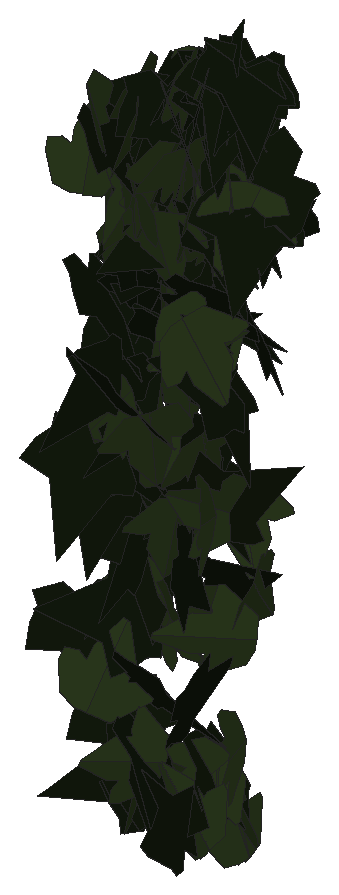
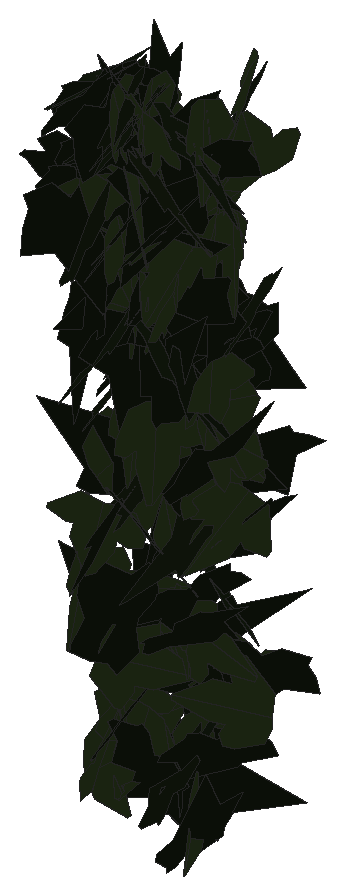
# SketchUp Ruby script. Lengths in inches.
U = 1.inch
M = Sketchup.active_model
def pt(a) = Geom::Point3d.new(a.map { |v| v * U })
def face(e, loops, mat)
  f = e.add_face(loops[0].map { |a| pt(a) })
  loops[1..].each { |l| e.add_face(l.map { |a| pt(a) }).erase! }
  f.material = f.back_material = mat if mat
  f
end
# faces: each face lists its corners as indices into pts; further lists are holes
def faces(e, pts, list, mat = nil) = list.each { |f| face(e, (f[0].is_a?(Array) ? f : [f]).map { |l| l.map { |i| pts[i] } }, mat) }
# xy, xz, yz: faces in a plane at the given z, y or x. An outline is a flat list of corners, or four numbers for a rectangle; further outlines are holes
def ring(l) = l.size == 4 ? [[l[0], l[1]], [l[2], l[1]], [l[2], l[3]], [l[0], l[3]]] : l.each_slice(2).to_a
def flat(e, list, mat, &to3) = list.each { |f| face(e, (f[0].is_a?(Array) ? f : [f]).map { |l| ring(l).map { |u, v| to3.(u, v) } }, mat) }
def xy(e, z, list, mat = nil) = flat(e, list, mat) { |x, y| [x, y, z] }
def xz(e, y, list, mat = nil) = flat(e, list, mat) { |x, z| [x, y, z] }
def yz(e, x, list, mat = nil) = flat(e, list, mat) { |y, z| [x, y, z] }
def lines(e, pts, list) = list.each { |a, b| e.add_line(pt(pts[a]), pt(pts[b])) }
# prism: a flat outline (further loops are holes) pulled along v
def prism(e, loops, v, mat = nil)
  f = face(e, loops, mat); d = Geom::Vector3d.new(v.map { |x| x * U })
  f.pushpull(f.normal.samedirection?(d) ? d.length : -d.length)
end
def box(e, o, s, mat = nil) = prism(e, [[o, [o[0] + s[0], o[1], o[2]], [o[0] + s[0], o[1] + s[1], o[2]], [o[0], o[1] + s[1], o[2]]]], [0, 0, s[2]], mat)
def at(x, y, z, deg = 0) = Geom::Transformation.translation(pt([x, y, z])) * Geom::Transformation.rotation(ORIGIN, Z_AXIS, deg.degrees)
def axes(o, x, y, z) = Geom::Transformation.new([*x, 0, *y, 0, *z, 0, *pt(o).to_a, 1])
def part(name) = M.definitions.add(name)
# library, detail: a bought-in or finely detailed component or shape, given as its bounding box
def library(name, o, s) = part(name).tap { |d| box(d.entities, o, s) }
def detail(e, o, s) = box(e.add_group.entities, o, s)
def put(e, d, t, mat = nil) = e.add_instance(d, t).tap { |i| i.material = mat if mat }
def group(e, t, mat = nil) = e.add_group.tap { |g| g.transformation = t; g.material = mat if mat }.entities
root = M.entities
M.materials.add("efeu1").color = [18, 25, 13]
M.materials.add("efeu2").color = [43, 57, 29]
c1 = part("ivyleaf_9")
p = [[1.54,2.16,1.25],[1.36,2.04,1.19],[-0.21,0.99,0.68],[-0.71,1.11,0.82],[-0.85,0.86,0.67],[-0.8,0.17,0.21],
  [-0.9,-0.01,0.1],[-0.67,-0.16,-0.02],[-0.08,-0.08,-0.05],[-0.03,-0.6,-0.4],[0.65,-0.88,-0.66],[0.83,-0.6,-0.49],
  [1.29,-0.42,-0.43],[1.8125,-0.07,-0.26],[1.21,0.44,0.15]]
faces(c1.entities,p,[[0,1,2,3,4,5,6,7,8,9,10,11,12,13,14]],"efeu1")
c2 = part("ivyleaf_10")
p = [[0,0.5,-0.03],[-0.0625,2.02,-0.43],[-0.19,2.01,-0.46],[-0.54,1.05,-0.29],[-0.52,0.625,-0.18],[-0.83,0.76,-0.28],
  [-1.16,0.64,-0.33],[-1.15,0.33,-0.24],[-0.77,-0.39,0.02],[-0.3,-0.51,0.16],[0.04,-0.48,0.23],[-0.02,2.01,-0.4375],
  [-0.06,2.01,-0.43],[0.04,-0.49,0.23],[0.67,-0.49,0.14],[1.38,0.36,-0.2],[1.375,0.51,-0.24],[0.81,0.65,-0.19],
  [0.62,0.59,-0.15],[0.6,1.09,-0.28],[0.5,1.23,-0.31]]
faces(c2.entities,p,[[0,1,2,3,4,5,6,7,8,9,10],[11,12,0,13,14,15,16,17,18,19,20]],"efeu2")
put(root,c1,axes([38.62,221.91,229.58],[0.41285,-0.18874,0.20961],[0.19514,-0.07719,-0.45383],[0.20367,0.45653,0.00992]))
put(root,c1,axes([38.49,222.17,228.38],[-0.24735,-0.43365,-0.02777],[0.01571,0.02301,-0.49922],[0.43425,-0.24784,0.00224]))
put(root,c1,axes([38.86,222.24,229.68],[-0.01844,0.06405,-0.49554],[0.11887,-0.48108,-0.0666],[-0.48531,-0.12027,0.00252]))
put(root,c2,axes([40.45,221.91,223.74],[0.31496,0.01944,0.38785],[-0.3877,-0.01282,0.31548],[0.02221,-0.49946,0.007]))
put(root,c1,axes([40.11,221.92,223.42],[0.03225,-0.03661,0.49761],[-0.37092,0.33178,0.04845],[-0.33374,-0.37227,-0.00576]))
put(root,c2,axes([39.22,222.34,224.11],[0.01236,0.1741,0.46855],[-0.03449,-0.46728,0.17454],[0.49866,-0.03664,0.00046]))
put(root,c1,axes([40.32,221.65,225.4375],[0.05676,0.20175,0.45396],[0.14531,0.43018,-0.20935],[-0.47504,0.1557,-0.0098]))
put(root,c2,axes([38.68,222.01,233.44],[-0.2553,0.42468,0.06682],[-0.04323,0.05196,-0.49541],[-0.42773,-0.25874,0.01019]))
put(root,c2,axes([39.48,222.1,229.09],[-0.25058,-0.4274,-0.06735],[0.0357,0.05715,-0.49544],[0.4312,-0.2531,0.00187]))
put(root,c2,axes([40.47,221.99,228.17],[0.19964,-0.24767,-0.38575],[-0.22067,0.31686,-0.31765],[0.40181,0.29708,0.01721]))
put(root,c2,axes([38.65,222.02,225.03],[0.39129,0.2317,-0.20786],[0.17364,0.11464,0.45465],[0.25834,-0.42799,0.00925]))
put(root,c1,axes([38.625,222.14,233.13],[0.33685,-0.31897,-0.18653],[-0.13671,0.12691,-0.4639],[0.34328,0.36353,-0.00172]))
put(root,c1,axes([39.06,222.51,224.19],[0.10296,-0.37972,0.30857],[0.08328,-0.29712,-0.39342],[0.48215,0.13241,0.00207]))
put(root,c2,axes([40.19,222.02,230.62],[0.20376,0.40619,0.20856],[0.08145,0.19238,-0.45426],[-0.44928,0.21909,0.01223]))
put(root,c2,axes([38.89,222.2,229.21],[0.35444,-0.19467,-0.29406],[-0.25425,0.14786,-0.40434],[0.24439,0.43616,0.00583]))
put(root,c1,axes([39.08,222.25,225.3125],[0.43114,-0.15485,0.20036],[0.1939,-0.05256,-0.45786],[0.16286,0.4725,0.01473]))
put(root,c2,axes([38.43,222.09,232.3125],[0.20213,0.41477,-0.19264],[0.07314,0.17858,0.46126],[0.45143,-0.21465,0.01152]))
put(root,c1,axes([39.53,222.66,232.94],[0.00322,-0.14379,0.47887],[0.14859,-0.45697,-0.13822],[0.4774,0.1432,0.03979]))
put(root,c2,axes([39.14,222.24,232.16],[-0.383,0.16339,0.2768],[-0.2783,0.04687,-0.41274],[-0.16082,-0.47022,0.05504]))
put(root,c2,axes([40.28,222.4,224.36],[0.39749,0.01003,-0.30315],[-0.30331,0.00841,-0.39741],[-0.00287,0.49983,0.01278]))
put(root,c1,axes([38.8,222.74,225.92],[-0.0306,-0.37999,-0.32352],[-0.01036,-0.32358,0.38104],[-0.49896,0.03003,0.01193]))
put(root,c1,axes([40.16,222.77,224.13],[-0.07141,-0.34765,0.35219],[-0.01375,-0.35431,-0.35253],[0.49468,-0.06003,0.04104]))
put(root,c2,axes([38.7,222.74,231.8],[-0.11246,-0.10863,0.47492],[0.23369,-0.43971,-0.04524],[0.42748,0.2118,0.14967]))
put(root,c2,axes([40.25,222.72,227.83],[-0.15186,-0.18622,-0.43847],[-0.2673,-0.34763,0.24022],[-0.39432,0.30737,0.00602]))
put(root,c1,axes([38.91,222.76,228.37],[-0.05128,0.01975,-0.49697],[0.08392,-0.4921,-0.02821],[-0.49023,-0.0863,0.04716]))
put(root,c2,axes([40.64,222.33,224.83],[0.27703,-0.28765,-0.30085],[-0.20353,0.22163,-0.39932],[0.36309,0.34371,0.0057]))
put(root,c1,axes([38.98,222.75,223.83],[-0.09241,-0.10733,-0.47952],[-0.1271,-0.4661,0.12882],[-0.47466,0.1457,0.05887]))
put(root,c2,axes([39.22,222.7,232.49],[0.03959,-0.43857,0.23682],[0.0717,-0.23009,-0.43809],[0.49325,0.06864,0.04467]))
put(root,c2,axes([39.33,222.43,231.73],[-0.47963,-0.1324,-0.04929],[0.04759,0.01284,-0.49756],[0.13302,-0.48198,0.00029]))
put(root,c1,axes([38.17,222.55,230.57],[0.30655,-0.39259,-0.04357],[-0.02168,0.03834,-0.49806],[0.39441,0.30725,0.00648]))
put(root,c2,axes([38.87,222.47,232.99],[0.19451,-0.42779,-0.17077],[-0.05219,0.16371,-0.46955],[0.45765,0.20049,0.01903]))
put(root,c1,axes([38,222.6,225.82],[-0.18784,-0.33209,-0.32316],[0.20844,0.25087,-0.37897],[0.41384,-0.27709,0.0442]))
put(root,c1,axes([38.86,222.66,226.95],[-0.42469,0.15832,-0.21112],[0.19522,-0.08064,-0.45319],[-0.17755,-0.46737,0.00667]))
put(root,c2,axes([40.22,222.84,226.01],[0.03854,0.04543,0.49644],[-0.28015,-0.40988,0.05926],[0.41235,-0.28273,-0.00614]))
put(root,c1,axes([38.15,222.87,227.64],[-0.04836,-0.48816,0.09674],[-0.01484,-0.09574,-0.49052],[0.49743,-0.05031,-0.00523]))
put(root,c1,axes([39.73,222.37,227.16],[0.20414,-0.11676,-0.44124],[-0.38034,0.2237,-0.23516],[0.25232,0.43166,0.00251]))
put(root,c2,axes([39.46,222.66,227.625],[-0.19801,-0.45567,0.0562],[-0.0135,-0.0554,-0.49674],[0.45892,-0.19824,0.00964]))
put(root,c2,axes([39.93,222.56,224.18],[-0.49142,0.07733,-0.05026],[0.04991,-0.00615,-0.49746],[-0.07756,-0.49395,-0.00167]))
put(root,c2,axes([39.57,222.65,232.66],[-0.10962,-0.48639,-0.03748],[0.01254,0.03559,-0.49857],[0.48767,-0.11025,0.0044]))
put(root,c2,axes([40.48,222.62,223.33],[-0.06185,0.49433,0.04255],[0.00517,-0.04224,0.49819],[0.49613,0.06207,0.00012]))
put(root,c2,axes([39.65,222.33,230.3],[-0.03849,-0.06343,-0.49446],[0.3307,0.36786,-0.07293],[0.37304,-0.33265,0.01364]))
put(root,c1,axes([38.92,222.83,232.41],[-0.46571,-0.04493,-0.17633],[0.17802,-0.01226,-0.46707],[0.03765,-0.49783,0.02741]))
put(root,c2,axes([39.12,222.62,228.22],[0.34343,0.01928,0.36288],[-0.36239,-0.01893,0.34397],[0.027,-0.49927,0.00097]))
put(root,c2,axes([40.51,222.61,223.42],[-0.27535,0.13116,-0.39621],[-0.35646,0.17297,0.30498],[0.21707,0.45042,-0.00175]))
put(root,c1,axes([39.38,222.53,230.31],[0.41566,0.2219,-0.16729],[-0.14569,-0.08231,-0.47117],[-0.23665,0.44044,-0.00377]))
put(root,c1,axes([39.9,223.0625,229.39],[0.12378,-0.45609,-0.16327],[0.05656,-0.15376,0.4724],[-0.48112,-0.13542,0.01353]))
put(root,c2,axes([39.87,222.64,228.72],[-0.0734,-0.46758,-0.1612],[0.03111,0.15828,-0.47327],[0.4936,-0.0795,0.00586]))
put(root,c1,axes([38.52,222.83,224.57],[-0.12638,-0.42652,-0.22827],[0.09732,0.20869,-0.44382],[0.47387,-0.15661,0.03027]))
put(root,c2,axes([38.79,222.49,231.62],[-0.19087,-0.2219,-0.40538],[0.25354,0.31641,-0.29258],[0.38638,-0.31724,-0.00826]))
put(root,c1,axes([39.97,222.63,227.8],[-0.0263,0.01334,0.49913],[0.49468,-0.06716,0.02786],[0.06779,0.49529,-0.00967]))
put(root,c2,axes([38.26,223.03,229.02],[0.06525,-0.39132,0.30432],[0.03314,-0.30282,-0.39649],[0.49461,0.07191,-0.01358]))
put(root,c1,axes([39.21,223.16,231.4],[-0.32274,-0.24371,0.29402],[-0.1154,-0.30471,-0.37925],[0.36404,-0.31266,0.14043]))
put(root,c2,axes([39.77,223.01,230.29],[0.18907,0.21224,-0.41135],[-0.28798,-0.29394,-0.28402],[-0.36238,0.34432,0.01109]))
put(root,c2,axes([38.45,222.68,231.62],[-0.38433,0.23883,0.21273],[-0.21824,0.04729,-0.44736],[-0.23381,-0.43672,0.06789]))
put(root,c1,axes([39.5,222.85,224.03],[-0.12961,-0.10189,-0.47204],[0.42836,0.20139,-0.16109],[0.22295,-0.44616,0.03509]))
put(root,c1,axes([38.52,222.92,229.97],[0.01312,-0.47866,-0.14392],[0.0147,0.14428,-0.47851],[0.49961,0.00832,0.01786]))
put(root,c2,axes([38.99,222.96,225.82],[0.00788,-0.05639,0.49675],[0.49074,-0.09398,-0.01845],[0.09545,0.48784,0.05387]))
put(root,c1,axes([38.97,223.13,223.86],[0.11787,-0.34687,0.34028],[0.15633,-0.30446,-0.36451],[0.46007,0.19232,0.03669]))
put(root,c2,axes([38.81,222.96,226.07],[-0.14378,0.02675,0.47813],[-0.4641,-0.13086,-0.13224],[0.11806,-0.48183,0.06246]))
put(root,c2,axes([38.875,222.6875,223.6],[0.06569,-0.31628,-0.38164],[-0.0574,0.37753,-0.32276],[0.49233,0.08621,0.01329]))
put(root,c1,axes([39.48,223.13,233.36],[-0.23341,0.11728,-0.42634],[0.37913,-0.19501,-0.26121],[-0.22755,-0.44521,0.0021]))
put(root,c1,axes([39.45,222.78,230.6],[0.4629,0.01903,0.18806],[0.18753,0.01597,-0.46322],[-0.02364,0.49938,0.00764]))
put(root,c1,axes([40.3,223.17,232.06],[-0.26999,-0.40651,-0.10889],[0.0746,0.0811,-0.48771],[0.41418,-0.2796,0.01686]))
put(root,c1,axes([38.9375,222.92,230.96],[0.10994,0.39803,-0.28193],[-0.08736,-0.26826,-0.4128],[-0.47988,0.14002,0.01056]))
put(root,c1,axes([38.97,223.08,233.21],[-0.00645,-0.46677,-0.17913],[-0.00431,0.17919,-0.46677],[0.49994,-0.00447,-0.00634]))
put(root,c2,axes([39.5625,222.8,231.96],[0.15931,-0.35367,-0.3155],[-0.06175,0.31452,-0.38375],[0.4699,0.16123,0.05653]))
put(root,c2,axes([37.94,222.85,225.19],[-0.02387,-0.06104,0.49569],[0.42164,0.2635,0.05275],[-0.26767,0.42052,0.0389]))
put(root,c2,axes([40.29,223.08,232.06],[0.41054,0.22704,-0.17294],[-0.15679,-0.07375,-0.46902],[-0.23848,0.43933,0.01064]))
put(root,c1,axes([39.56,223.16,231.65],[0.20956,-0.45397,0.00013],[0.02202,0.01002,-0.49941],[0.45343,0.20932,0.0242]))
put(root,c1,axes([39.69,223.21,229.36],[0.20053,-0.45584,0.04473],[0.01419,-0.04263,-0.49798],[0.45781,0.20099,-0.00416]))
put(root,c2,axes([38.58,222.95,233.25],[0.02581,-0.46054,-0.19297],[-0.02219,0.19198,-0.46114],[0.49884,0.03237,-0.01053]))
put(root,c2,axes([38.31,223.17,228.56],[-0.16801,-0.45577,0.11851],[0.00836,-0.1287,-0.48308],[0.47085,-0.16034,0.05086]))
put(root,c2,axes([40.03,223.17,232],[-0.16886,-0.03288,0.46947],[-0.41432,-0.22618,-0.16487],[0.22321,-0.4447,0.04914]))
put(root,c1,axes([38.78,222.94,230.58],[0.24103,0.35705,-0.25381],[-0.14125,-0.21088,-0.43079],[-0.41467,0.27936,-0.00079]))
put(root,c1,axes([38.52,223.12,232.93],[-0.14518,-0.38557,-0.28329],[0.13248,0.25208,-0.41098],[0.45975,-0.1944,0.02897]))
put(root,c1,axes([39.59,223.07,231.09],[-0.09093,0.04353,0.48973],[-0.45988,0.16863,-0.10038],[-0.1739,-0.46869,0.00937]))
put(root,c1,axes([38.79,222.97,223.09],[-0.19634,-0.34061,0.30892],[0.1535,0.26809,0.39315],[-0.43346,0.24922,-0.0007]))
put(root,c1,axes([39.04,223.22,233.02],[-0.38397,-0.14166,-0.28723],[0.27812,0.07483,-0.40871],[0.15879,-0.47364,0.02133]))
put(root,c1,axes([38.62,223.27,226.83],[-0.09332,-0.48374,-0.08536],[0.0153,0.08398,-0.49266],[0.49098,-0.09456,-0.00088]))
put(root,c2,axes([39.5,223.26,232.72],[0.30438,-0.13706,0.37225],[0.36423,-0.0893,-0.3307],[0.15713,0.47248,0.04548]))
put(root,c2,axes([38.84,223.3,230.84],[-0.06198,0.40604,-0.28511],[0.05434,-0.28004,-0.41064],[-0.49316,-0.08189,-0.00942]))
put(root,c1,axes([38.89,223.05,233.125],[-0.31671,0.37985,0.07354],[-0.06421,0.04211,-0.49407],[-0.38154,-0.32239,0.02211]))
put(root,c2,axes([38.21,223.28,229.9],[-0.02693,-0.49653,0.05223],[0.18094,-0.05846,-0.46243],[0.46533,-0.00601,0.18283]))
put(root,c1,axes([38.64,223.01,231.02],[-0.02924,-0.12676,-0.48278],[0.17659,0.44971,-0.12877],[0.46686,-0.17804,0.01847]))
put(root,c2,axes([38.08,223,228.05],[-0.25602,-0.28035,-0.32536],[0.21499,0.24424,-0.37964],[0.37179,-0.33429,-0.00452]))
put(root,c1,axes([38.63,223.29,230.1],[-0.3251,0.26577,-0.27143],[0.21456,-0.16635,-0.41987],[-0.31349,-0.38947,-0.00588]))
put(root,c2,axes([39.61,223.27,231.42],[0.02773,-0.49809,0.03368],[0.01151,-0.03308,-0.49877],[0.4991,0.02844,0.00963]))
put(root,c2,axes([39.19,223.21,233.45],[0.12144,-0.48366,-0.03643],[0.12343,0.06714,-0.47985],[0.46906,0.10755,0.1357]))
put(root,c1,axes([39.58,223.01,232.91],[-0.38126,0.28998,0.14336],[0.11417,-0.08669,0.47901],[0.30266,0.39799,-0.00011]))
put(root,c1,axes([39.4,223.15,231.9],[0.29083,-0.33974,-0.2236],[-0.10698,0.2013,-0.44501],[0.39239,0.30669,0.0444]))
put(root,c1,axes([38.36,223.52,228.44],[-0.13332,0.10452,0.47043],[-0.32191,-0.38254,-0.00624],[0.35861,-0.30453,0.16929]))
put(root,c1,axes([39.82,223.52,233.59],[-0.23194,-0.44097,-0.04183],[0.0094,0.04231,-0.49812],[0.44285,-0.23186,-0.01134]))
put(root,c2,axes([39.52,223.18,230.89],[0.35432,-0.31528,-0.15828],[-0.00877,0.21639,-0.45066],[0.35267,0.32214,0.14781]))
put(root,c1,axes([40.54,223.51,232.36],[-0.45822,-0.14385,0.13908],[-0.13545,-0.0328,-0.48018],[0.14727,-0.47774,-0.00891]))
put(root,c1,axes([38.96,223.1,232.35],[0.44878,0.18559,-0.11898],[-0.11001,-0.04532,-0.48564],[-0.19104,0.46206,0.00016]))
put(root,c1,axes([39.78,223.57,232.8125],[-0.29409,-0.40362,-0.02452],[0.03926,0.00168,-0.49845],[0.40245,-0.29511,0.03071]))
put(root,c1,axes([39.08,223.45,228.3125],[0.27556,-0.41161,0.06814],[0.02947,-0.06225,-0.49523],[0.41617,0.27695,-0.01004]))
put(root,c1,axes([39.34,223.59,233.13],[0.06861,-0.48005,0.12185],[0.01235,-0.12132,-0.4849],[0.49512,0.06955,-0.00479]))
put(root,c1,axes([39.8,223.59,233.63],[-0.01218,-0.48823,0.10718],[0.16525,-0.10511,-0.46005],[0.47175,0.02422,0.16391]))
put(root,c1,axes([39.46,223.07,229.9],[0.10534,0.48835,0.02048],[0.00378,0.02013,-0.49958],[-0.48876,0.10541,0.00055]))
put(root,c2,axes([39.45,223.58,225.75],[0.10546,0.12789,-0.47172],[-0.41561,-0.23047,-0.1554],[-0.25718,0.42489,0.0577]))
put(root,c1,axes([39.51,223.4375,227.79],[-0.4677,0.17654,-0.00935],[0.00876,-0.00326,-0.49991],[-0.17657,-0.46778,-0.00004]))
put(root,c2,axes([38.73,223.21,231.37],[0.23564,0.37395,0.23375],[0.09682,0.21469,-0.44106],[-0.43023,0.25313,0.02877]))
put(root,c1,axes([39.6,223.58,233.3],[-0.085,0.26781,-0.41359],[0.07869,-0.40693,-0.27967],[-0.4864,-0.11264,0.02703]))
put(root,c1,axes([40.22,223.23,230.25],[0.28987,0.00576,-0.40736],[-0.40606,0.0447,-0.28831],[0.03309,0.49796,0.03059]))
put(root,c1,axes([38.76,223.51,231.97],[0.17233,-0.46088,-0.08881],[0.00947,0.098,-0.49021],[0.46927,0.16728,0.0425]))
put(root,c1,axes([39.58,223.35,227.71],[0.24534,-0.34684,-0.26365],[-0.14799,0.21825,-0.42481],[0.40977,0.28648,0.00444]))
put(root,c1,axes([39.83,223.76,231.4],[0.10152,-0.3146,0.37513],[0.09909,-0.36198,-0.33039],[0.47945,0.14143,-0.01115]))
put(root,c2,axes([40.22,223.23,226.54],[0.02816,-0.37549,-0.32896],[-0.01559,0.32866,-0.37649],[0.49896,0.03146,0.0068]))
put(root,c1,axes([40.32,223.4,231.7],[0.0102,0.4277,-0.25879],[0.00412,-0.2589,-0.42773],[-0.49988,0.0066,-0.00881]))
put(root,c2,axes([39.39,223.61,233.44],[0.14286,-0.45034,0.16367],[0.13393,-0.12645,-0.46483],[0.46006,0.17665,0.0845]))
put(root,c1,axes([38.97,223.42,230.26],[-0.38442,0.31954,-0.0107],[0.00825,-0.0068,-0.49989],[-0.31962,-0.38451,-0.00004]))
put(root,c1,axes([39.29,223.5,226.23],[0.4209,0.14596,-0.22703],[0.21512,0.07258,0.44548],[0.163,-0.47268,-0.0017]))
put(root,c1,axes([38.96,223.49,229.58],[0.17434,-0.26813,0.38434],[-0.2292,0.30889,0.31946],[-0.40875,-0.28756,-0.01521]))
put(root,c1,axes([38.34,223.84,226.62],[-0.27691,-0.39053,0.14425],[-0.01421,-0.16429,-0.47203],[0.41607,-0.26552,0.07989]))
put(root,c2,axes([39.79,223.46,227.5625],[0.43769,0.19617,0.14122],[0.12466,0.06708,-0.47954],[-0.20709,0.45499,0.00981]))
put(root,c2,axes([39,223.58,233.34],[0.46064,-0.11589,0.15613],[0.15384,-0.02831,-0.4749],[0.11892,0.48556,0.00958]))
put(root,c1,axes([39.45,223.32,230.44],[0.37973,-0.18556,-0.26715],[-0.17248,0.23331,-0.40721],[0.27579,0.40141,0.11318]))
put(root,c1,axes([39.17,223.65,233.29],[0.24931,-0.43083,0.04727],[0.04427,-0.02893,-0.4972],[0.43115,0.25209,0.02372]))
put(root,c1,axes([38.34,223.38,227.86],[0.4338,-0.20129,-0.14595],[-0.08262,0.16012,-0.46641],[0.2345,0.42877,0.10566]))
put(root,c2,axes([38.92,223.49,229.17],[-0.24402,-0.43121,-0.06715],[0.02426,0.06341,-0.49537],[0.43573,-0.24502,-0.01002]))
put(root,c2,axes([39.27,223.53,232.35],[0.23077,-0.42966,-0.11015],[-0.05763,0.09407,-0.48768],[0.4398,0.23778,-0.00611]))
put(root,c1,axes([39.35,223.53,233.51],[0.40301,-0.29246,-0.04533],[-0.03518,0.02869,-0.49793],[0.29385,0.40453,0.00254]))
put(root,c1,axes([39.04,223.625,232.78],[-0.44116,0.20878,-0.10859],[0.08783,-0.06797,-0.48751],[-0.21832,-0.44921,0.0233]))
put(root,c1,axes([39.79,223.8,233.55],[-0.03565,-0.49838,0.01856],[-0.00444,-0.01829,-0.49965],[0.49871,-0.03579,-0.00312]))
